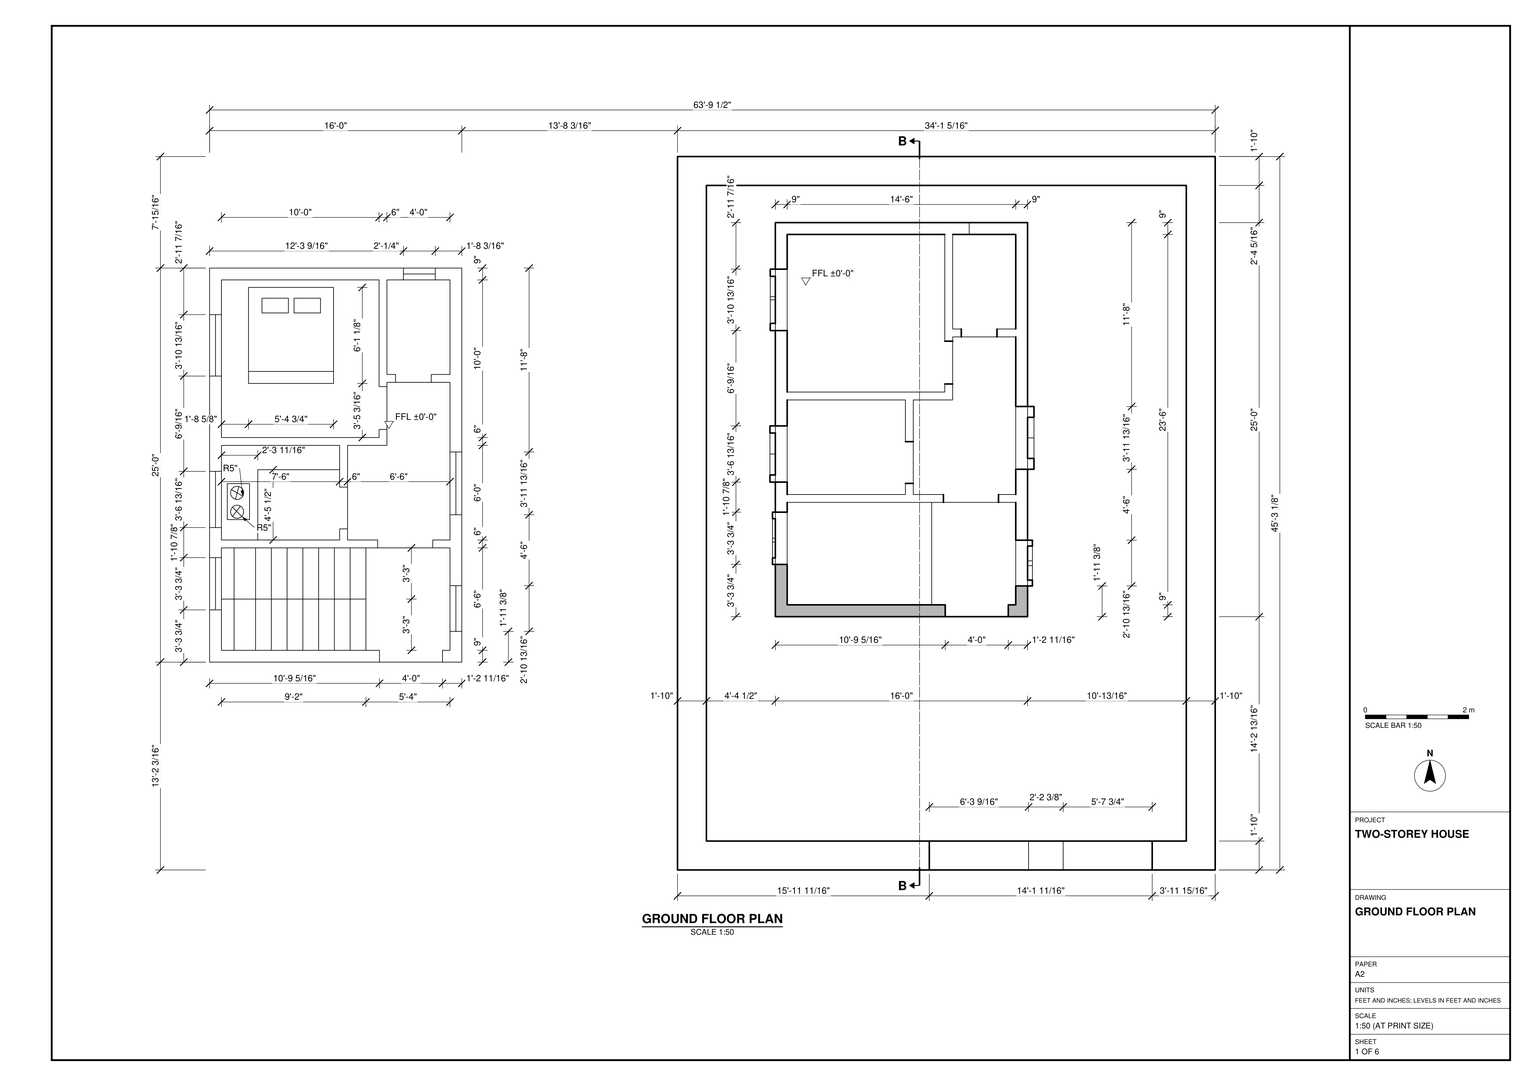
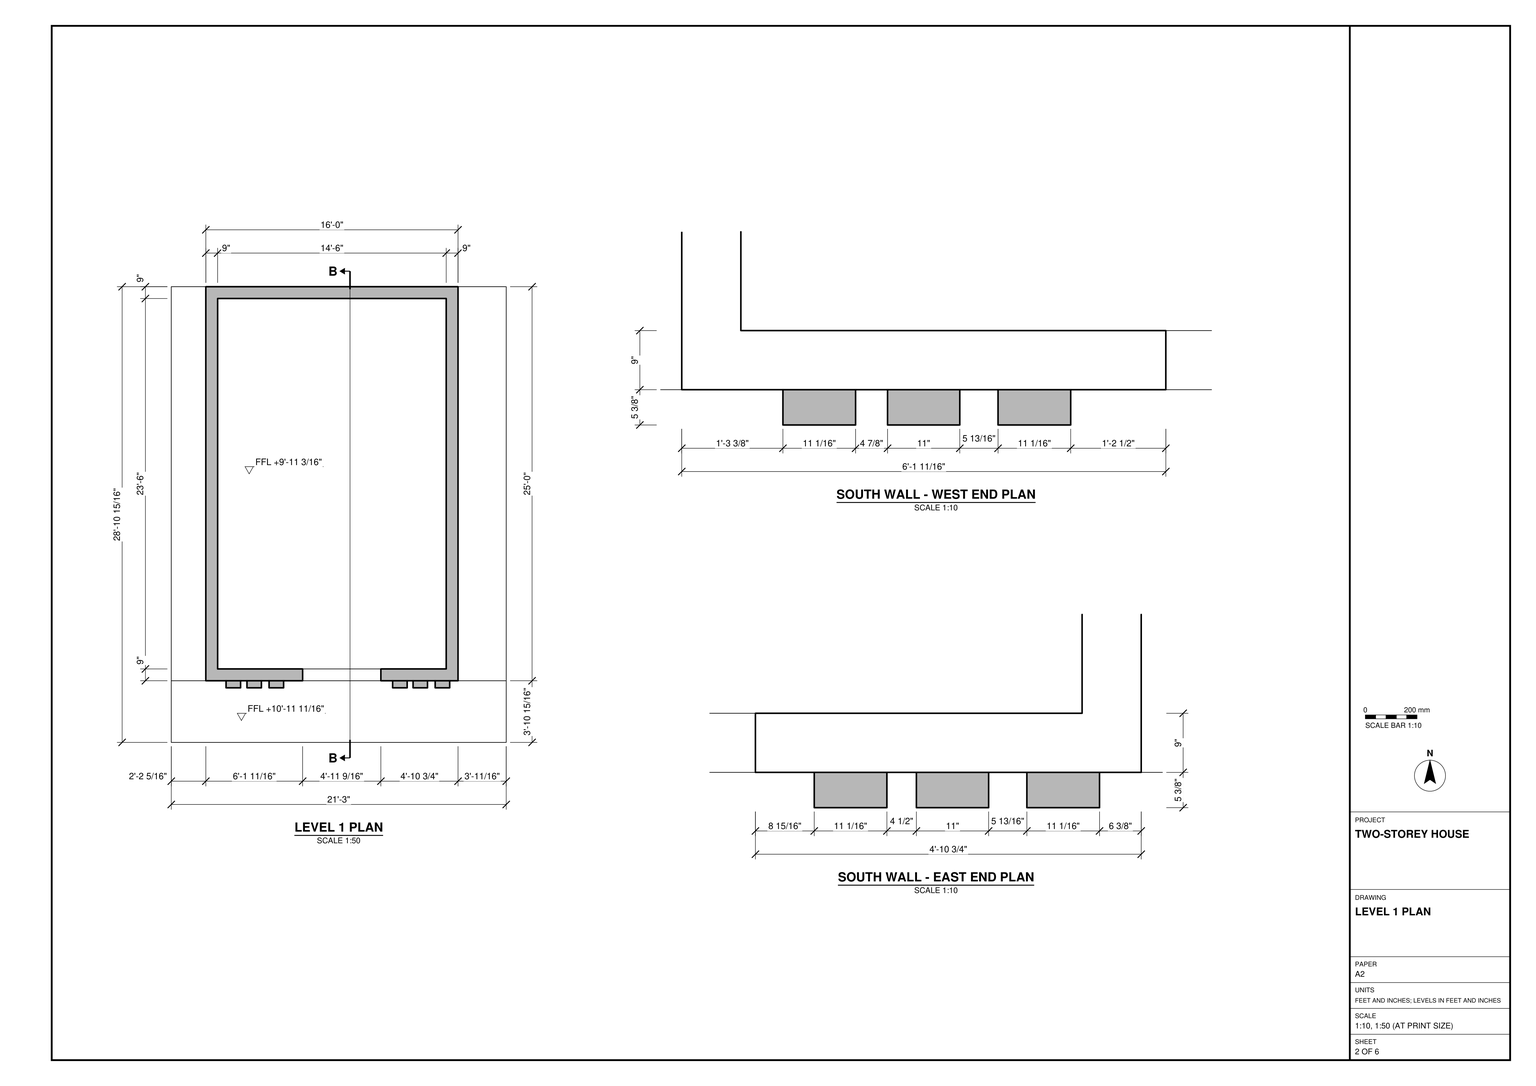
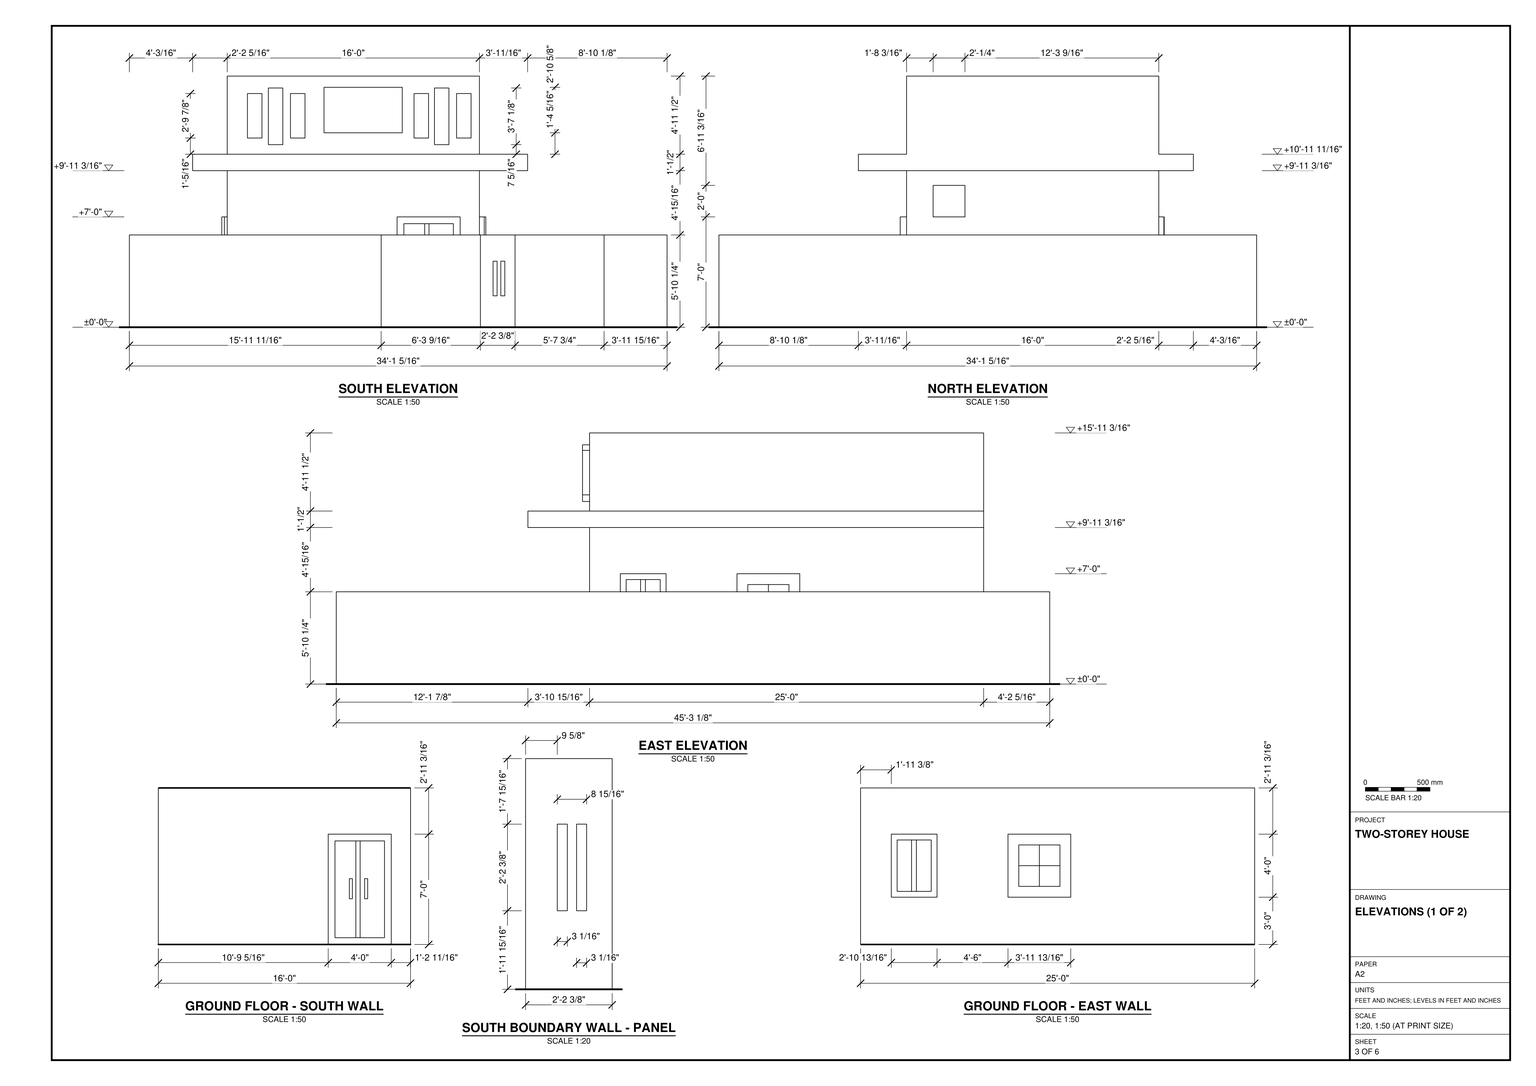
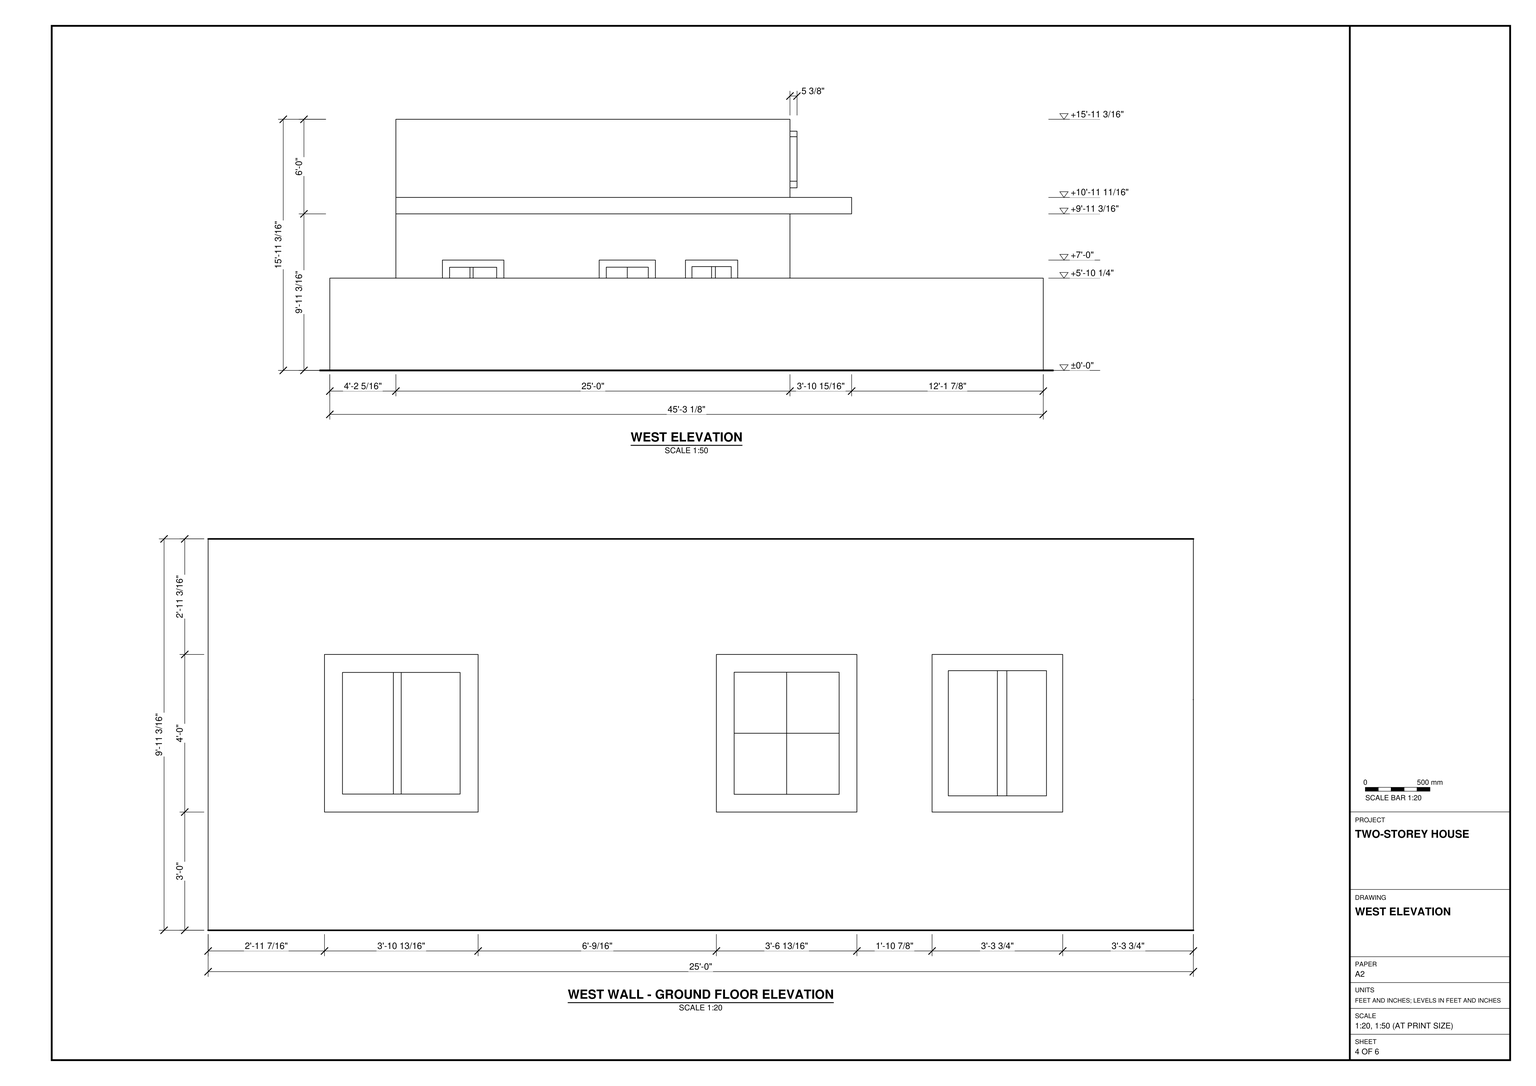
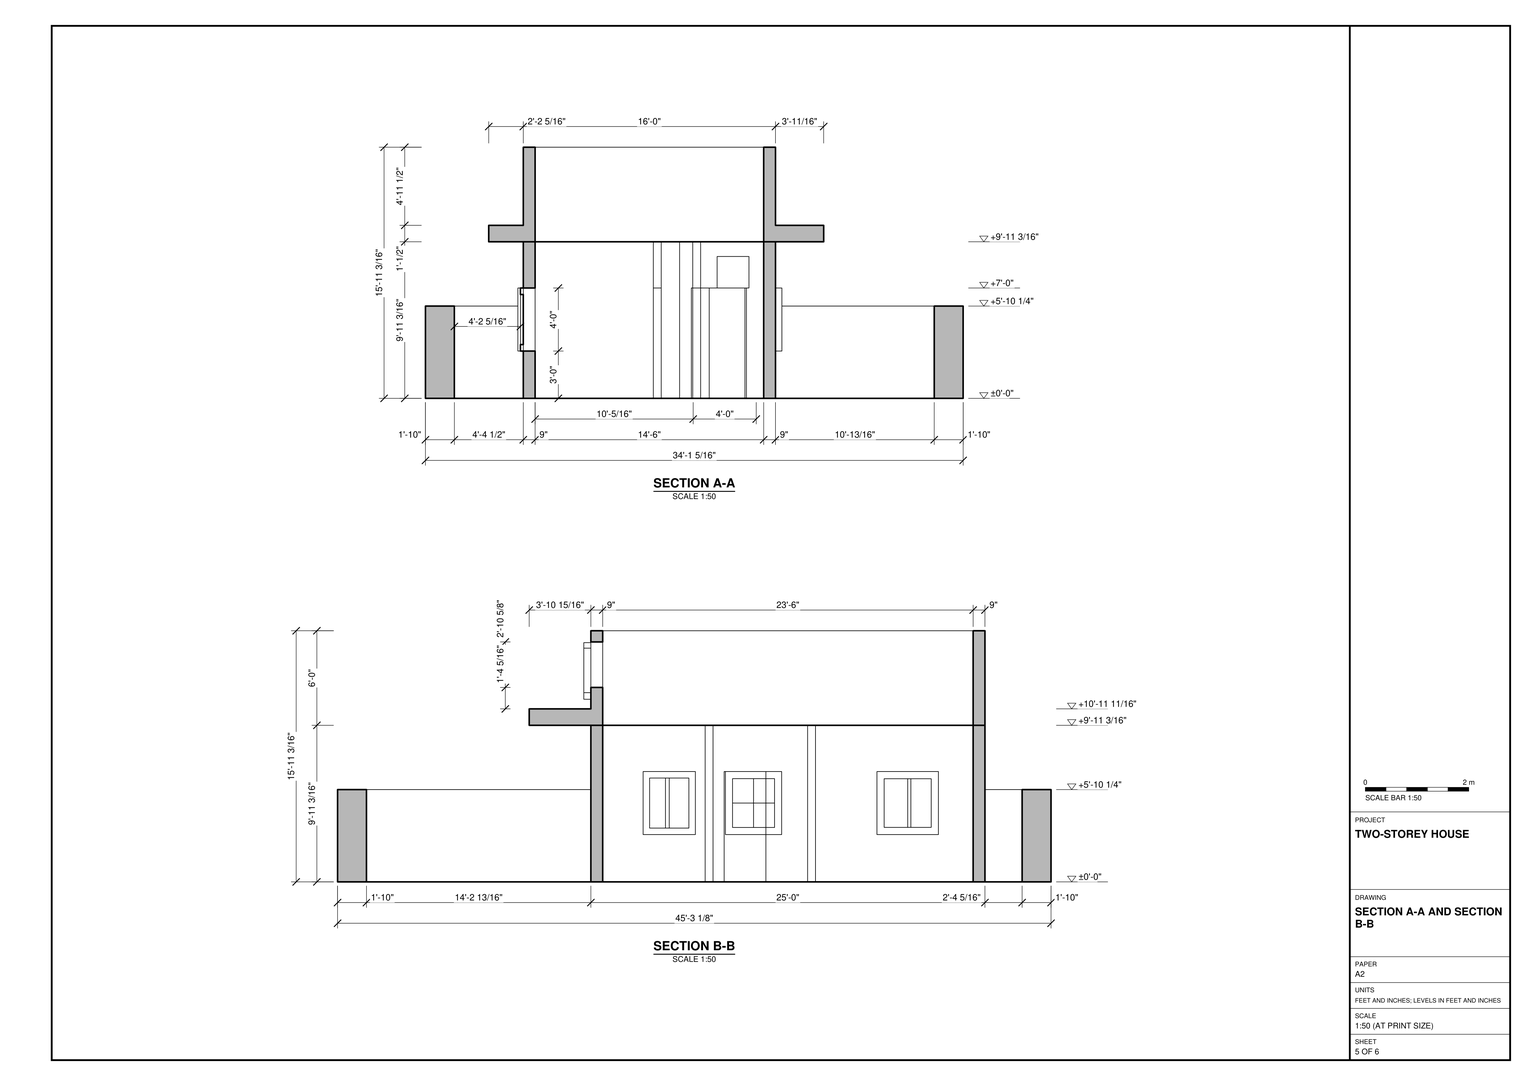
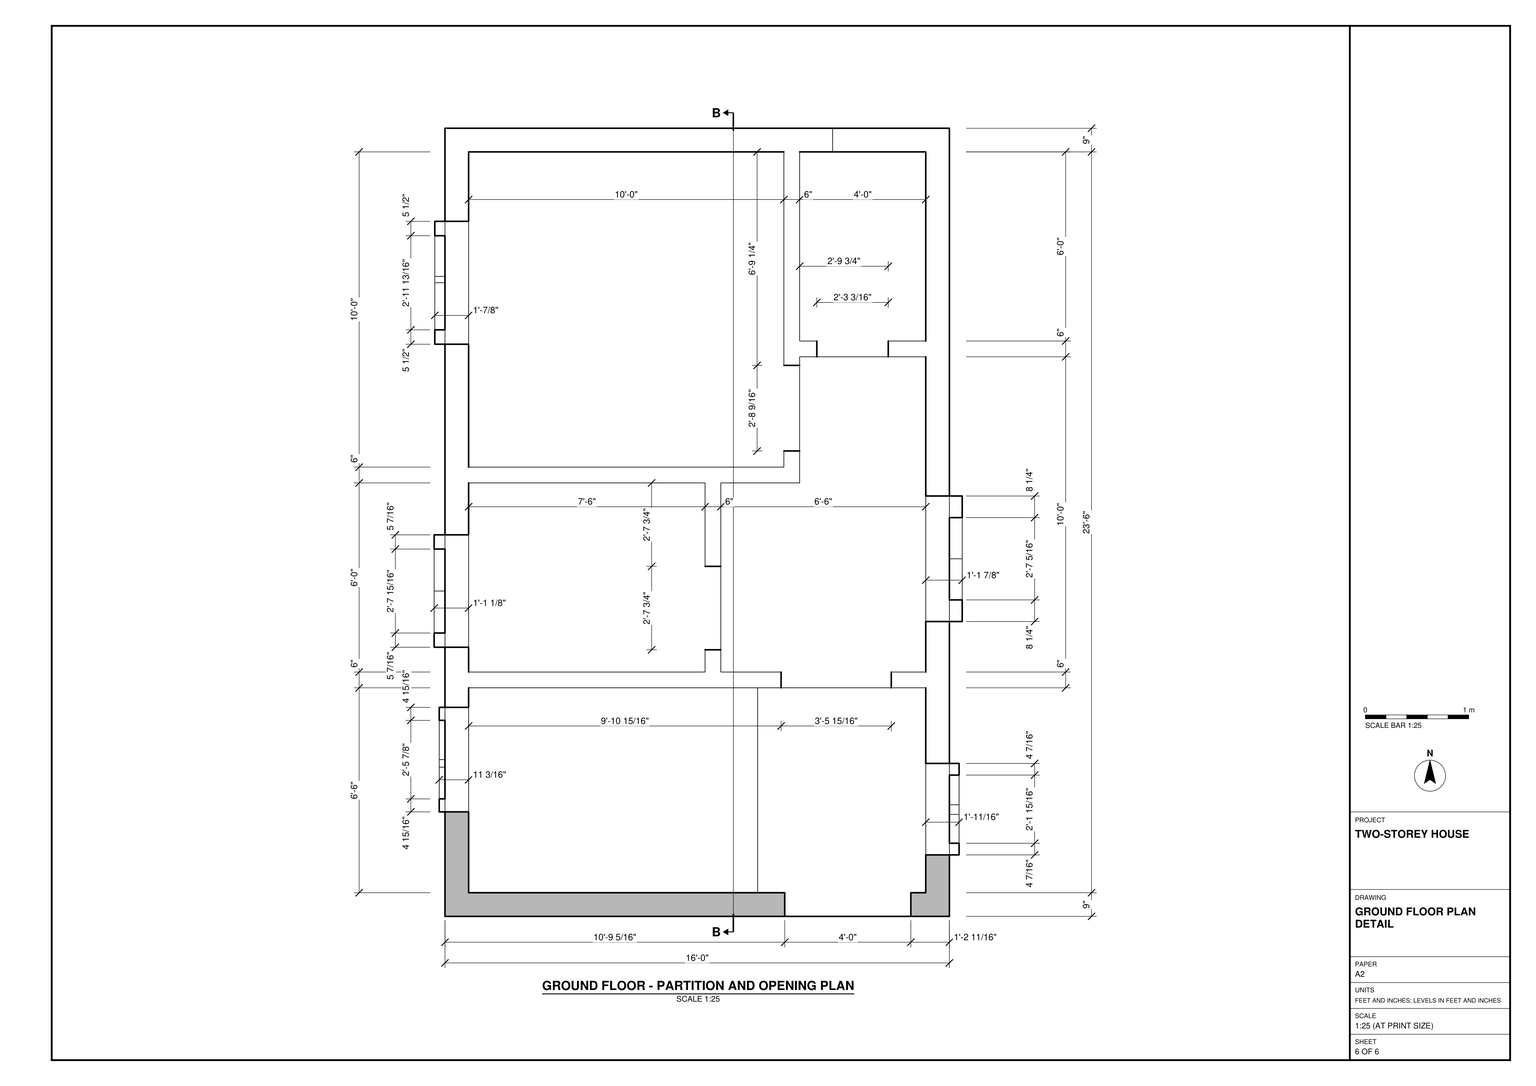
Build the two-storey house in SketchUp from task_files/diagram_01.pdf. Work in feet and inches. The complete model, including the separate furnished ground-floor layout west of the plot, measures 63'-9 1/2" east to west, 45'-3 1/8" north to south and 15'-11 3/16" high. Set the ground floor at ±0'-0" and the upper level at +9'-11 3/16".

Use the ground-floor plan to position the house within the rectangular boundary wall, leaving the larger yard to the south. Include the entrance panels in the south boundary and the double door in the south wall of the house. Follow the drawn wall thicknesses, room divisions, doorways and window positions. Model the flat roof slab with its unequal projections beyond the walls below. Use the upper-level plan and elevations to place the walls above the slab and the narrow projecting panels on either side of the south opening.

Keep the furnished ground-floor layout in its drawn position outside the boundary. Include its partitions, bed, kitchen counter with cooktop, and stair flights. Model shell elements such as walls, slabs and roof, and each furniture or joinery piece, as separate groups or components; use components for repeated parts. Decor and loose items may be any suitable library components. Save one SketchUp model as output_files/two_storey_house_walled_plot_and_furnished_ground_floor.skp.

# SketchUp Ruby script. Lengths in inches.
U = 1.inch
M = Sketchup.active_model
def pt(a) = Geom::Point3d.new(a.map { |v| v * U })
def face(e, loops, mat)
  f = e.add_face(loops[0].map { |a| pt(a) })
  loops[1..].each { |l| e.add_face(l.map { |a| pt(a) }).erase! }
  f.material = f.back_material = mat if mat
  f
end
# faces: each face lists its corners as indices into pts; further lists are holes
def faces(e, pts, list, mat = nil) = list.each { |f| face(e, (f[0].is_a?(Array) ? f : [f]).map { |l| l.map { |i| pts[i] } }, mat) }
# xy, xz, yz: faces in a plane at the given z, y or x. An outline is a flat list of corners, or four numbers for a rectangle; further outlines are holes
def ring(l) = l.size == 4 ? [[l[0], l[1]], [l[2], l[1]], [l[2], l[3]], [l[0], l[3]]] : l.each_slice(2).to_a
def flat(e, list, mat, &to3) = list.each { |f| face(e, (f[0].is_a?(Array) ? f : [f]).map { |l| ring(l).map { |u, v| to3.(u, v) } }, mat) }
def xy(e, z, list, mat = nil) = flat(e, list, mat) { |x, y| [x, y, z] }
def xz(e, y, list, mat = nil) = flat(e, list, mat) { |x, z| [x, y, z] }
def yz(e, x, list, mat = nil) = flat(e, list, mat) { |y, z| [x, y, z] }
def lines(e, pts, list) = list.each { |a, b| e.add_line(pt(pts[a]), pt(pts[b])) }
# prism: a flat outline (further loops are holes) pulled along v
def prism(e, loops, v, mat = nil)
  f = face(e, loops, mat); d = Geom::Vector3d.new(v.map { |x| x * U })
  f.pushpull(f.normal.samedirection?(d) ? d.length : -d.length)
end
def box(e, o, s, mat = nil) = prism(e, [[o, [o[0] + s[0], o[1], o[2]], [o[0] + s[0], o[1] + s[1], o[2]], [o[0], o[1] + s[1], o[2]]]], [0, 0, s[2]], mat)
def at(x, y, z, deg = 0) = Geom::Transformation.translation(pt([x, y, z])) * Geom::Transformation.rotation(ORIGIN, Z_AXIS, deg.degrees)
def axes(o, x, y, z) = Geom::Transformation.new([*x, 0, *y, 0, *z, 0, *pt(o).to_a, 1])
def part(name) = M.definitions.add(name)
# library, detail: a bought-in or finely detailed component or shape, given as its bounding box
def library(name, o, s) = part(name).tap { |d| box(d.entities, o, s) }
def detail(e, o, s) = box(e.add_group.entities, o, s)
def put(e, d, t, mat = nil) = e.add_instance(d, t).tap { |i| i.material = mat if mat }
def group(e, t, mat = nil) = e.add_group.tap { |g| g.transformation = t; g.material = mat if mat }.entities
root = M.entities
M.materials.add("[Blinds Cloth Horizontal]").color = [192, 163, 85]
M.materials.add("[Blinds Roman Hobbled Blue]").color = [81, 82, 87]
M.materials.add("[Blinds Wood Light]").color = [155, 100, 14]
M.materials.add("[Cladding Siding Tan]").color = [162, 126, 95]
M.materials.add("[Cladding Siding White]").color = [207, 207, 207]
M.materials.add("[Formica Beige]").color = [211, 187, 149]
M.materials.add("[Formica Blue]").color = [71, 97, 152]
M.materials.add("[Formica Graystone]").color = [149, 146, 135]
M.materials.add("[Formica Laminate Dark]").color = [50, 53, 60]
M.materials.add("[Formica Laminate Light]").color = [213, 189, 164]
M.materials.add("[Formica Speckled Grey]").color = [94, 105, 111]
M.materials.add("[Terrazzo Tile Light]").color = [219, 217, 210]
M.materials.add("[Translucent Glass Blue]").color = [100, 149, 237]
M.materials["[Translucent Glass Blue]"].alpha = 0.5
M.materials.add("[Water Light Blue]").color = [102, 169, 251]
M.materials.add("[Window Covering 01]").color = [169, 163, 146]
M.materials.add("[Wood Bamboo]").color = [177, 105, 43]
M.materials.add("[Wood Floor Light]").color = [204, 176, 127]
M.materials.add("[Wood Veneer 01]").color = [120, 70, 37]
xy(root,0,[[356.21,0,356.21,543.125,765.52,543.125,765.52,0,717.57,0,717.57,22,743.52,22,743.52,521.125,378.21,521.125,378.21,22,547.89,22,547.89,0],[547.89,0,623.43,22],[623.43,0,649.8,22],[649.8,0,717.57,22],[0,158.21,129.32,158.21,129.32,167.21,9,167.21,9,197.99,0,197.99],
  [129.32,158.21,177.32,158.21,177.32,167.21,183,167.21,183,245.21,119,245.21,119,167.21,129.32,167.21],[177.32,158.21,192,158.21,192,181.61,183,181.61,183,167.21,177.32,167.21],[9,167.21,18.625,206.21],[18.625,167.21,35,206.21],[35,167.21,47,206.21],
  [47,167.21,59,206.21],[59,167.21,71,206.21],[71,167.21,83,206.21],[83,167.21,95,206.21],[95,167.21,107,206.21],
  [107,167.21,119,206.21],[183,181.61,187.5,216.43],[187.5,181.61,192,216.43],[430.6875,192.83,560.01,192.83,560.01,201.83,439.6875,201.83,439.6875,232.61,430.6875,232.61],[608.01,192.83,622.6875,192.83,622.6875,251.04,613.6875,251.04,613.6875,201.83,608.01,201.83],
  [0,197.99,4.5,237.77],[4.5,197.99,9,237.77],[9,206.21,18.625,245.21],[18.625,206.21,35,245.21],[35,206.21,47,245.21],
  [47,206.21,59,245.21],[59,206.21,71,245.21],[71,206.21,83,245.21],[83,206.21,95,245.21],[95,206.21,107,245.21],
  [107,206.21,119,245.21],[183,216.43,192,216.43,192,270.44,183,270.44,183,251.21,169.88,251.21,169.88,245.21,183,245.21],[430.6875,232.61,439.6875,232.61,439.6875,279.83,558.63,279.83,558.63,285.83,535.6875,285.83,535.6875,294.3,529.6875,294.3,529.6875,285.83,439.6875,285.83,439.6875,295.27,430.6875,295.27],[0,237.77,9,237.77,9,245.21,127.94,245.21,127.94,251.21,105,251.21,105,259.68,99,259.68,99,251.21,9,251.21,9,260.66,0,260.66],[127.94,245.21,169.88,245.21,169.88,251.21,183,251.21,183,371.21,135,371.21,135,323.21,105,323.21,105,251.21,127.94,251.21],
  [613.6875,251.04,622.6875,251.04,622.6875,352.84,613.6875,352.84,613.6875,285.83,600.57,285.83,600.57,279.83,613.6875,279.83],[[9,251.21,36.68,251.21,36.68,304.71,99,304.71,99,323.21,9,323.21],[13.46,266.73,30.4,294.14]],[36.68,251.21,99,251.21,99,259.68,105,259.68,105,291.45,99,291.45,99,304.71,36.68,304.71],[0,260.66,4.5,303.45],[4.5,260.66,9,303.45],
  [[13.46,266.73,30.4,294.14],[20.95,282.07,19.65,282.24,18.45,282.74,17.41,283.54,16.61,284.57,16.12,285.78,15.95,287.07,16.12,288.37,16.61,289.57,17.41,290.61,18.45,291.4,19.65,291.9,20.95,292.07,22.24,291.9,23.45,291.4,24.48,290.61,25.28,289.57,25.77,288.37,25.95,287.07,25.77,285.78,25.28,284.57,24.48,283.54,23.45,282.74,22.24,282.24],[20.95,267.7,19.65,267.87,18.45,268.37,17.41,269.16,16.61,270.2,16.12,271.4,15.95,272.7,16.12,273.99,16.61,275.2,17.41,276.23,18.45,277.03,19.65,277.53,20.95,277.7,22.24,277.53,23.45,277.03,24.48,276.23,25.28,275.2,25.77,273.99,25.95,272.7,25.77,271.4,25.28,270.2,24.48,269.16,23.45,268.37,22.24,267.87]],[20.95,267.7,22.24,267.87,23.45,268.37,24.48,269.16,20.48,273.16,17.41,269.16,18.45,268.37,19.65,267.87],[17.41,269.16,20.48,273.16,17.41,276.23,16.61,275.2,16.12,273.99,15.95,272.7,16.12,271.4,16.61,270.2],[24.48,269.16,25.28,270.2,25.77,271.4,25.95,272.7,25.77,273.99,25.28,275.2,24.48,276.23,23.45,277.03,20.48,273.16],[183,270.44,187.5,318.22],
  [187.5,270.44,192,318.22],[20.48,273.16,23.45,277.03,22.24,277.53,20.95,277.7,19.65,277.53,18.45,277.03,17.41,276.23],[20.95,282.07,22.24,282.24,23.45,282.74,24.48,283.54,25.28,284.57,20.95,287.07,19.65,282.24],[19.65,282.24,20.95,287.07,16.61,289.57,16.12,288.37,15.95,287.07,16.12,285.78,16.61,284.57,17.41,283.54,18.45,282.74],[25.28,284.57,25.77,285.78,25.95,287.07,25.77,288.37,25.28,289.57,24.48,290.61,23.45,291.4,22.24,291.9,20.95,287.07],
  [20.95,287.07,22.24,291.9,20.95,292.07,19.65,291.9,18.45,291.4,17.41,290.61,16.61,289.57],[99,291.45,105,291.45,105,323.21,135,323.21,135,335.37,129,335.37,129,329.21,9,329.21,9,376,0,376,0,303.45,9,303.45,9,323.21,99,323.21],[430.6875,295.27,439.6875,295.27,439.6875,357.83,529.6875,357.83,529.6875,326.0625,535.6875,326.0625,535.6875,357.83,565.6875,357.83,565.6875,369.98,559.6875,369.98,559.6875,363.83,439.6875,363.83,439.6875,410.61,430.6875,410.61],[183,318.22,192,318.22,192,458.21,171.8,458.21,171.8,449.21,183,449.21,183,377.21,168.73,377.21,168.73,371.21,183,371.21],[[9,329.21,129,329.21,129,335.37,135,335.37,135,367.95,129,367.95,129,449.21,9,449.21],[29.625,370.38,94.375,443.5]],
  [613.6875,352.84,622.6875,352.84,622.6875,492.83,578.24,492.83,578.24,483.83,613.6875,483.83,613.6875,411.83,599.41,411.83,599.41,405.83,613.6875,405.83],[129,367.95,135,367.95,135,371.21,141.54,371.21,141.54,377.21,135,377.21,135,449.21,147.55,449.21,147.55,458.21,0,458.21,0,422.78,9,422.78,9,449.21,129,449.21],[29.625,370.38,94.375,379.52],[141.54,371.21,168.73,371.21,168.73,377.21,183,377.21,183,449.21,135,449.21,135,377.21,141.54,377.21],[0,376,4.5,422.78],
  [4.5,376,9,422.78],[[29.625,379.52,94.375,443.5],[39.87,424.04,59.99,435.29],[64.31,424.04,84.43,435.29]],[559.6875,402.5625,565.6875,402.5625,565.6875,405.83,572.23,405.83,572.23,411.83,565.6875,411.83,565.6875,483.83,578.24,483.83,578.24,492.83,430.6875,492.83,430.6875,410.61,439.6875,410.61,439.6875,483.83,559.6875,483.83],[39.87,424.04,59.99,435.29],[64.31,424.04,84.43,435.29],
  [147.55,449.21,171.8,453.71],[147.55,453.71,171.8,458.21]])
xy(root,0,[[[378.21,22,743.52,521.125],[430.6875,192.83,622.6875,492.83]],[560.01,192.83,608.01,192.83,608.01,201.83,613.6875,201.83,613.6875,279.83,549.6875,279.83,549.6875,201.83,560.01,201.83],[439.6875,201.83,549.6875,279.83],[558.63,279.83,600.57,279.83,600.57,285.83,613.6875,285.83,613.6875,405.83,565.6875,405.83,565.6875,357.83,535.6875,357.83,535.6875,285.83,558.63,285.83],[439.6875,285.83,529.6875,285.83,529.6875,294.3,535.6875,294.3,535.6875,326.0625,529.6875,326.0625,529.6875,357.83,439.6875,357.83],
  [439.6875,363.83,559.6875,363.83,559.6875,369.98,565.6875,369.98,565.6875,402.5625,559.6875,402.5625,559.6875,483.83,439.6875,483.83],[572.23,405.83,599.41,405.83,599.41,411.83,613.6875,411.83,613.6875,483.83,565.6875,483.83,565.6875,411.83,572.23,411.83]],"[Terrazzo Tile Light]")
xy(root,36,[[428.5,232.61,430.6875,272.38],[430.6875,232.61,439.6875,272.38],[430.6875,295.27,439.6875,338.0625],[613.6875,305.06,622.6875,352.84],[430.6875,410.61,439.6875,457.4]])
xy(root,36,[[622.6875,216.23,626.375,251.04],[426.8125,410.61,430.6875,457.4]],"[Wood Bamboo]")
xy(root,36,[[426.5625,295.27,430.6875,338.0625],[622.6875,305.06,627.5625,352.84]],"[Wood Veneer 01]")
xy(root,40.43,[[622.6875,220.66,626.375,231.64],[622.6875,231.64,626.375,235.32],[622.6875,235.32,626.375,246.61]],"[Wood Bamboo]")
xy(root,40.94,[[428.5,237.55,430.6875,249.62],[428.5,249.62,430.6875,252.5],[428.5,252.5,430.6875,267.44]])
xy(root,41.41,[[426.5625,300.68,430.6875,316.67],[426.5625,316.67,430.6875,332.65]],"[Wood Veneer 01]")
xy(root,41.48,[[426.8125,416.09,430.6875,434.03],[426.8125,434.03,430.6875,436.42],[426.8125,436.42,430.6875,451.91]],"[Wood Bamboo]")
xy(root,44.23,[[622.6875,313.28,627.5625,328.95],[622.6875,328.95,627.5625,344.61]],"[Wood Veneer 01]")
xy(root,70.25,[[547.89,0,623.43,22],[649.8,0,717.57,22]],"[Formica Laminate Dark]")
xy(root,70.25,[[356.21,0,547.89,0,547.89,22,378.21,22,378.21,521.125,743.52,521.125,743.52,22,717.57,22,717.57,0,765.52,0,765.52,543.125,356.21,543.125]],"[Formica Laminate Light]")
xy(root,70.25,[[623.43,0,649.8,22]],"[Formica Speckled Grey]")
xy(root,75.77,[[622.6875,313.28,627.5625,328.95],[622.6875,328.95,627.5625,344.61]],"[Wood Veneer 01]")
xy(root,78.52,[[426.8125,416.09,430.6875,434.03],[426.8125,434.03,430.6875,436.42],[426.8125,436.42,430.6875,451.91]],"[Wood Bamboo]")
xy(root,78.59,[[426.5625,300.68,430.6875,316.67],[426.5625,316.67,430.6875,332.65]],"[Wood Veneer 01]")
xy(root,79.06,[[428.5,237.55,430.6875,249.62],[428.5,249.62,430.6875,252.5],[428.5,252.5,430.6875,267.44]])
xy(root,79.57,[[622.6875,220.66,626.375,231.64],[622.6875,231.64,626.375,235.32],[622.6875,235.32,626.375,246.61]],"[Wood Bamboo]")
xy(root,84,[[560.01,192.83,608.01,201.83],[428.5,232.61,430.6875,272.38],[430.6875,232.61,439.6875,272.38],[558.63,279.83,600.57,285.83],[529.6875,294.3,535.6875,326.0625],
  [430.6875,295.27,439.6875,338.0625],[613.6875,305.06,622.6875,352.84],[559.6875,369.98,565.6875,402.5625],[572.23,405.83,599.41,411.83],[430.6875,410.61,439.6875,457.4],
  [578.24,483.83,602.49,492.83]])
xy(root,84,[[622.6875,216.23,626.375,251.04],[426.8125,410.61,430.6875,457.4]],"[Wood Bamboo]")
xy(root,84,[[426.5625,295.27,430.6875,338.0625],[622.6875,305.06,627.5625,352.84]],"[Wood Veneer 01]")
xy(root,108,[[578.24,483.83,602.49,492.83]])
xy(root,119.1875,[[[430.6875,192.83,622.6875,492.83],[439.6875,201.83,613.6875,483.83]],[439.6875,201.83,613.6875,483.83]])
xy(root,119.1875,[[404.375,145.89,659.375,192.83],[404.375,192.83,430.6875,492.83],[622.6875,192.83,659.375,492.83]],"[Formica Graystone]")
xy(root,131.7,[[404.375,145.89,659.375,192.83],[404.375,192.83,430.6875,492.83],[622.6875,192.83,659.375,492.83]],"[Formica Graystone]")
xy(root,139,[[462.02,187.45,473.02,192.83],[588.46,187.45,599.46,192.83]])
xy(root,144.05,[[446.09,187.45,457.15,192.83],[478.84,187.45,489.9,192.83],[572.9,187.45,583.97,192.83],[605.28,187.45,616.34,192.83]])
xy(root,148.03,[[504.39,192.83,563.95,201.83]],"[Formica Beige]")
xy(root,177.92,[[446.09,187.45,457.15,192.83],[478.84,187.45,489.9,192.83],[572.9,187.45,583.97,192.83],[605.28,187.45,616.34,192.83]],"[Formica Blue]")
xy(root,182.13,[[462.02,187.45,473.02,192.83],[588.46,187.45,599.46,192.83]],"[Formica Blue]")
xy(root,182.66,[[504.39,192.83,563.95,201.83]],"[Formica Beige]")
xy(root,191.1875,[[430.6875,192.83,439.6875,192.83,439.6875,483.83,613.6875,483.83,613.6875,192.83,622.6875,192.83,622.6875,492.83,430.6875,492.83],[439.6875,192.83,613.6875,201.83]])
xz(root,0,[[633.08,23.92,636.14,50.3],[638.96,23.92,642.02,50.3]],"[Formica Beige]")
xz(root,0,[[547.89,0,623.43,70.25],[649.8,0,717.57,70.25]],"[Formica Laminate Dark]")
xz(root,0,[[356.21,0,547.89,70.25],[717.57,0,765.52,70.25]],"[Formica Laminate Light]")
xz(root,0,[[[623.43,0,649.8,70.25],[638.96,23.92,642.02,50.3],[633.08,23.92,636.14,50.3]]],"[Formica Speckled Grey]")
xz(root,22,[[547.89,0,623.43,70.25],[649.8,0,717.57,70.25]],"[Formica Laminate Dark]")
xz(root,22,[[378.21,0,547.89,70.25],[717.57,0,743.52,70.25]],"[Formica Laminate Light]")
xz(root,22,[[623.43,0,649.8,70.25]],"[Formica Speckled Grey]")
xz(root,145.89,[[404.375,119.1875,659.375,131.7]],"[Formica Graystone]")
xz(root,187.45,[[462.02,139,473.02,182.13],[588.46,139,599.46,182.13],[446.09,144.05,457.15,177.92],[478.84,144.05,489.9,177.92],[572.9,144.05,583.97,177.92],
  [605.28,144.05,616.34,177.92]],"[Formica Blue]")
xz(root,192.83,[[462.02,139,473.02,182.13],[588.46,139,599.46,182.13],[446.09,144.05,457.15,177.92],[478.84,144.05,489.9,177.92],[572.9,144.05,583.97,177.92],
  [605.28,144.05,616.34,177.92]])
xz(root,192.83,[[430.6875,0,560.01,0,560.01,84,608.01,84,608.01,0,622.6875,0,622.6875,119.1875,430.6875,119.1875]],"[Cladding Siding Tan]")
xz(root,192.83,[[[430.6875,131.7,622.6875,191.1875],[504.39,148.03,563.95,182.66],[588.46,139,599.46,182.13],[462.02,139,473.02,182.13],[572.9,144.05,583.97,177.92],[605.28,144.05,616.34,177.92],[478.84,144.05,489.9,177.92],[446.09,144.05,457.15,177.92]]],"[Formica Beige]")
xz(root,201.83,[[[439.6875,119.1875,613.6875,191.1875],[504.39,148.03,563.95,182.66]]])
xz(root,201.83,[[439.6875,0,549.6875,119.1875],[549.6875,0,549.6875,119.1875,613.6875,119.1875,613.6875,0,608.01,0,608.01,84,560.01,84,560.01,0]],"[Formica Laminate Light]")
xz(root,216.23,[[613.6875,35.09,613.6875,85.56,622.6875,84,622.6875,36]])
xz(root,216.23,[[622.6875,36,626.375,84]],"[Wood Bamboo]")
xz(root,220.66,[[622.6875,40.43,626.375,79.57]],"[Wood Bamboo]")
xz(root,232.61,[[428.5,36,430.6875,84],[430.6875,36,439.6875,84]])
xz(root,237.55,[[428.5,40.94,430.6875,79.06]])
xz(root,246.61,[[622.6875,40.43,626.375,79.57]],"[Wood Bamboo]")
xz(root,251.04,[[613.6875,35.09,622.6875,36,622.6875,84,613.6875,85.56]])
xz(root,251.04,[[622.6875,36,626.375,84]],"[Wood Bamboo]")
xz(root,267.44,[[428.5,40.94,430.6875,79.06]])
xz(root,272.38,[[428.5,36,430.6875,84],[430.6875,36,439.6875,84]])
xz(root,294.3,[[529.6875,0,535.6875,84]])
xz(root,295.27,[[430.6875,36,439.6875,84]])
xz(root,295.27,[[426.5625,36,430.6875,84]],"[Wood Veneer 01]")
xz(root,300.68,[[426.5625,41.41,430.6875,60],[426.5625,60,430.6875,78.59]],"[Wood Veneer 01]")
xz(root,305.06,[[613.6875,36,622.6875,84]])
xz(root,305.06,[[622.6875,36,627.5625,84]],"[Wood Veneer 01]")
xz(root,313.28,[[622.6875,44.23,627.5625,60],[622.6875,60,627.5625,75.77]],"[Wood Veneer 01]")
xz(root,326.0625,[[529.6875,0,535.6875,84]])
xz(root,332.65,[[426.5625,41.41,430.6875,60],[426.5625,60,430.6875,78.59]],"[Wood Veneer 01]")
xz(root,338.0625,[[430.6875,36,439.6875,84]])
xz(root,338.0625,[[426.5625,36,430.6875,84]],"[Wood Veneer 01]")
xz(root,344.61,[[622.6875,44.23,627.5625,60],[622.6875,60,627.5625,75.77]],"[Wood Veneer 01]")
xz(root,352.84,[[613.6875,36,622.6875,84]])
xz(root,352.84,[[622.6875,36,627.5625,84]],"[Wood Veneer 01]")
xz(root,369.98,[[559.6875,0,565.6875,84]])
xz(root,402.5625,[[559.6875,0,565.6875,84]])
xz(root,410.61,[[430.6875,36,439.6875,84]])
xz(root,410.61,[[426.8125,36,430.6875,84]],"[Wood Bamboo]")
xz(root,416.09,[[426.8125,41.48,430.6875,78.52]],"[Wood Bamboo]")
xz(root,451.91,[[426.8125,41.48,430.6875,78.52]],"[Wood Bamboo]")
xz(root,457.4,[[430.6875,36,439.6875,84]])
xz(root,457.4,[[426.8125,36,430.6875,84]],"[Wood Bamboo]")
xz(root,483.83,[[439.6875,119.1875,613.6875,191.1875]])
xz(root,483.83,[[439.6875,0,559.6875,119.1875]],"[Formica Blue]")
xz(root,483.83,[[[565.6875,0,613.6875,119.1875],[578.24,84,602.49,108]]],"[Water Light Blue]")
xz(root,492.83,[[[430.6875,0,622.6875,119.1875],[578.24,84,602.49,108]]],"[Cladding Siding White]")
xz(root,492.83,[[404.375,119.1875,404.375,131.7,430.6875,131.7,430.6875,191.1875,622.6875,191.1875,622.6875,131.7,659.375,131.7,659.375,119.1875]],"[Formica Beige]")
xz(root,521.125,[[378.21,0,743.52,70.25]],"[Formica Laminate Light]")
xz(root,543.125,[[356.21,0,765.52,70.25]],"[Formica Laminate Light]")
yz(root,356.21,[[0,0,543.125,70.25]],"[Formica Laminate Light]")
yz(root,378.21,[[22,0,521.125,70.25]],"[Formica Laminate Light]")
yz(root,404.375,[[145.89,119.1875,492.83,131.7]],"[Formica Graystone]")
yz(root,426.5625,[[[295.27,36,338.0625,84],[300.68,41.41,332.65,78.59]]],"[Wood Veneer 01]")
yz(root,426.8125,[[[410.61,36,457.4,84],[416.09,41.48,451.91,78.52]]],"[Wood Bamboo]")
yz(root,428.5,[[[232.61,36,272.38,84],[237.55,40.94,267.44,79.06]]])
yz(root,430.6875,[[249.62,40.94,252.5,79.06]])
yz(root,430.6875,[[416.09,41.48,434.03,78.52],[436.42,41.48,451.91,78.52]],"[Blinds Roman Hobbled Blue]")
yz(root,430.6875,[[237.55,40.94,249.62,79.06],[252.5,40.94,267.44,79.06]],"[Blinds Wood Light]")
yz(root,430.6875,[[[192.83,0,492.83,119.1875],[410.61,36,457.4,84],[295.27,36,338.0625,84],[232.61,36,272.38,84]]],"[Cladding Siding White]")
yz(root,430.6875,[[192.83,131.7,492.83,191.1875]],"[Formica Beige]")
yz(root,430.6875,[[300.68,41.41,316.67,60],[316.67,41.41,332.65,60],[300.68,60,316.67,78.59],[316.67,60,332.65,78.59]],"[Translucent Glass Blue]")
yz(root,430.6875,[[434.03,41.48,436.42,78.52]],"[Wood Bamboo]")
yz(root,439.6875,[[201.83,119.1875,483.83,191.1875]])
yz(root,439.6875,[[[285.83,0,357.83,119.1875],[295.27,36,338.0625,84]]],"[Formica Beige]")
yz(root,439.6875,[[[363.83,0,483.83,119.1875],[410.61,36,457.4,84]]],"[Formica Blue]")
yz(root,439.6875,[[[201.83,0,279.83,119.1875],[232.61,36,272.38,84]]],"[Formica Laminate Light]")
yz(root,446.09,[[187.45,144.05,192.83,177.92]],"[Formica Blue]")
yz(root,457.15,[[187.45,144.05,192.83,177.92]],"[Formica Blue]")
yz(root,462.02,[[187.45,139,192.83,182.13]],"[Formica Blue]")
yz(root,473.02,[[187.45,139,192.83,182.13]],"[Formica Blue]")
yz(root,478.84,[[187.45,144.05,192.83,177.92]],"[Formica Blue]")
yz(root,489.9,[[187.45,144.05,192.83,177.92]],"[Formica Blue]")
yz(root,504.39,[[192.83,148.03,201.83,182.66]],"[Formica Beige]")
yz(root,547.89,[[0,0,22,70.25]])
yz(root,558.63,[[279.83,0,285.83,84]])
yz(root,560.01,[[192.83,0,201.83,84]])
yz(root,563.95,[[192.83,148.03,201.83,182.66]],"[Formica Beige]")
yz(root,572.23,[[405.83,0,411.83,84]])
yz(root,572.9,[[187.45,144.05,192.83,177.92]],"[Formica Blue]")
yz(root,578.24,[[483.83,84,492.83,108]])
yz(root,583.97,[[187.45,144.05,192.83,177.92]],"[Formica Blue]")
yz(root,588.46,[[187.45,139,192.83,182.13]],"[Formica Blue]")
yz(root,599.41,[[405.83,0,411.83,84]])
yz(root,599.46,[[187.45,139,192.83,182.13]],"[Formica Blue]")
yz(root,600.57,[[279.83,0,285.83,84]])
yz(root,602.49,[[483.83,84,492.83,108]])
yz(root,605.28,[[187.45,144.05,192.83,177.92]],"[Formica Blue]")
yz(root,608.01,[[192.83,0,201.83,84]])
yz(root,613.6875,[[[201.83,0,279.83,119.1875],[216.23,35.09,251.04,85.56]],[[285.83,0,405.83,119.1875],[305.06,36,352.84,84]],[201.83,119.1875,483.83,191.1875]])
yz(root,613.6875,[[411.83,0,483.83,119.1875]],"[Water Light Blue]")
yz(root,616.34,[[187.45,144.05,192.83,177.92]],"[Formica Blue]")
yz(root,622.6875,[[220.66,40.43,231.64,79.57],[235.32,40.43,246.61,79.57]],"[Blinds Cloth Horizontal]")
yz(root,622.6875,[[[192.83,0,492.83,119.1875],[305.06,36,352.84,84],[216.23,36,251.04,84]]],"[Cladding Siding White]")
yz(root,622.6875,[[192.83,131.7,492.83,191.1875]],"[Formica Beige]")
yz(root,622.6875,[[313.28,44.23,328.95,60],[328.95,44.23,344.61,60],[313.28,60,328.95,75.77],[328.95,60,344.61,75.77]],"[Window Covering 01]")
yz(root,622.6875,[[231.64,40.43,235.32,79.57]],"[Wood Bamboo]")
yz(root,626.375,[[[216.23,36,251.04,84],[220.66,40.43,246.61,79.57]]],"[Wood Bamboo]")
yz(root,627.5625,[[[305.06,36,352.84,84],[313.28,44.23,344.61,75.77]]],"[Wood Veneer 01]")
yz(root,659.375,[[145.89,119.1875,492.83,131.7]],"[Formica Graystone]")
yz(root,717.57,[[0,0,22,70.25]])
yz(root,743.52,[[22,0,521.125,70.25]],"[Formica Laminate Light]")
yz(root,765.52,[[0,0,543.125,70.25]],"[Formica Laminate Light]")
p = [[613.6875,216.23,35.09],[622.6875,216.23,36],[622.6875,251.04,36],[613.6875,251.04,35.09],[622.6875,216.23,84],[613.6875,216.23,85.56],
  [613.6875,251.04,85.56],[622.6875,251.04,84],[187.5,270.44,0],[187.5,270.22,0],[565.6875,405.83,0],[565.6875,405.83,119.1875],
  [565.6875,411.83,0],[565.6875,411.83,119.1875],[549.6875,279.83,0],[549.6875,279.83,119.1875],[535.6875,285.83,0],[535.6875,285.83,119.1875],
  [529.6875,285.83,0],[529.6875,285.83,119.1875],[529.6875,357.83,0],[529.6875,357.83,119.1875],[535.6875,357.83,0],[535.6875,357.83,119.1875],
  [565.6875,357.83,0],[565.6875,357.83,119.1875],[559.6875,363.83,0],[559.6875,363.83,119.1875]]
faces(root,p,[[0,1,2,3],[4,5,6,7]])
lines(root,p,[[8,9],[10,11],[12,13],[14,15],[16,17],[18,19],[20,21],[22,23],[24,25],[26,27]])
g1 = group(root,at(560.01,192.83,0))
xz(g1,0,[[[0,0,48,84],[5.16,5.16,42.84,78.84]],[21.03,5.16,24.3,78.84]],"[Wood Bamboo]")
xz(g1,0,[[16.09,34.81,18.41,50.12],[27.72,34.81,30.03,50.12]],"[Wood Floor Light]")
xz(g1,0,[[[5.16,5.16,21.03,78.84],[16.09,34.81,18.41,50.12]],[[24.3,5.16,42.84,78.84],[27.72,34.81,30.03,50.12]]],"[Wood Veneer 01]")
